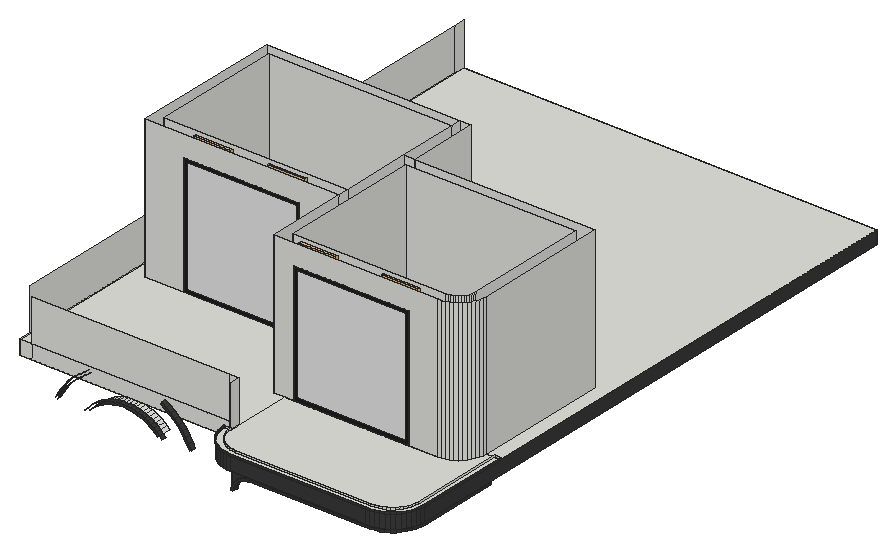
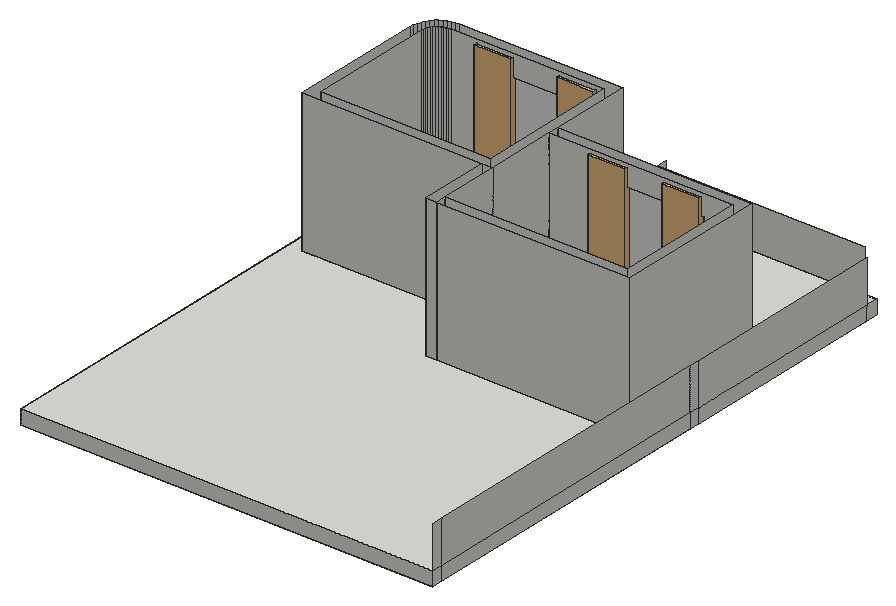
# SketchUp Ruby script. Lengths in inches.
U = 1.inch
M = Sketchup.active_model
def pt(a) = Geom::Point3d.new(a.map { |v| v * U })
def face(e, loops, mat)
  f = e.add_face(loops[0].map { |a| pt(a) })
  loops[1..].each { |l| e.add_face(l.map { |a| pt(a) }).erase! }
  f.material = f.back_material = mat if mat
  f
end
# faces: each face lists its corners as indices into pts; further lists are holes
def faces(e, pts, list, mat = nil) = list.each { |f| face(e, (f[0].is_a?(Array) ? f : [f]).map { |l| l.map { |i| pts[i] } }, mat) }
# xy, xz, yz: faces in a plane at the given z, y or x. An outline is a flat list of corners, or four numbers for a rectangle; further outlines are holes
def ring(l) = l.size == 4 ? [[l[0], l[1]], [l[2], l[1]], [l[2], l[3]], [l[0], l[3]]] : l.each_slice(2).to_a
def flat(e, list, mat, &to3) = list.each { |f| face(e, (f[0].is_a?(Array) ? f : [f]).map { |l| ring(l).map { |u, v| to3.(u, v) } }, mat) }
def xy(e, z, list, mat = nil) = flat(e, list, mat) { |x, y| [x, y, z] }
def xz(e, y, list, mat = nil) = flat(e, list, mat) { |x, z| [x, y, z] }
def yz(e, x, list, mat = nil) = flat(e, list, mat) { |y, z| [x, y, z] }
def lines(e, pts, list) = list.each { |a, b| e.add_line(pt(pts[a]), pt(pts[b])) }
# prism: a flat outline (further loops are holes) pulled along v
def prism(e, loops, v, mat = nil)
  f = face(e, loops, mat); d = Geom::Vector3d.new(v.map { |x| x * U })
  f.pushpull(f.normal.samedirection?(d) ? d.length : -d.length)
end
def box(e, o, s, mat = nil) = prism(e, [[o, [o[0] + s[0], o[1], o[2]], [o[0] + s[0], o[1] + s[1], o[2]], [o[0], o[1] + s[1], o[2]]]], [0, 0, s[2]], mat)
def at(x, y, z, deg = 0) = Geom::Transformation.translation(pt([x, y, z])) * Geom::Transformation.rotation(ORIGIN, Z_AXIS, deg.degrees)
def axes(o, x, y, z) = Geom::Transformation.new([*x, 0, *y, 0, *z, 0, *pt(o).to_a, 1])
def part(name) = M.definitions.add(name)
# library, detail: a bought-in or finely detailed component or shape, given as its bounding box
def library(name, o, s) = part(name).tap { |d| box(d.entities, o, s) }
def detail(e, o, s) = box(e.add_group.entities, o, s)
def put(e, d, t, mat = nil) = e.add_instance(d, t).tap { |i| i.material = mat if mat }
def group(e, t, mat = nil) = e.add_group.tap { |g| g.transformation = t; g.material = mat if mat }.entities
root = M.entities
M.materials.add("[Color M07]").color = [58, 58, 58]
M.materials.add("[Color M08]").color = [30, 30, 30]
M.materials.add("[Mirror 02]").color = [229, 229, 229]
c1 = library("Curtains 004",[-15.59,-2.26,0],[31.18,4.52,116.91])
xy(root,238.1,[[217.25,0,219.1875,4.75]])
xy(root,250.0625,[[233.71,0,233.71,4.75,331.6,4.75,334.94,4.79,338.01,5.25,340.98,6.125,343.8125,7.39,346.45,9.02,348.84,10.99,350.9375,13.27,352.71,15.82,354.125,18.57,355.16,21.5,355.78,24.53,356,27.76,356,96.75,360.75,96.75,360.75,27.6,360.5,23.89,359.74,20.22,358.5,16.69,356.79,13.36,354.65,10.29,352.11,7.54,349.22,5.15,346.04,3.18,342.625,1.65,339.03,0.6,335.33,0.05,331.63,0]],"[Color M07]")
xy(root,251.99,[[233.4,0,233.48,0.75]],"[Color M07]")
xy(root,252,[[216.6875,0.75,213.16,0.98,209.7,1.67,206.36,2.81,203.1875,4.37,200.25,6.33,197.6,8.66,195.27,11.3125,193.3,14.25,191.74,17.42,190.61,20.76,189.92,24.23,189.6875,27.75,189.99,24.2,190.75,20.73,191.95,17.375,193.57,14.21,195.58,11.27,197.96,8.625,200.66,6.3,203.63,4.35,206.83,2.79,210.21,1.67,213.7,0.98,217.25,0.75],[217.25,0.75,217.25,6.3,214.48,6.66,211.76,7.33,209.15,8.32,206.66,9.6,204.34,11.16,202.22,12.98,200.32,15.03,198.68,17.29,197.31,19.73,196.23,22.31,195.46,24.99,195,27.75,189.6875,27.75,189.99,24.2,190.75,20.73,191.95,17.375,193.57,14.21,195.58,11.27,197.96,8.625,200.66,6.3,203.63,4.35,206.83,2.79,210.21,1.67,213.7,0.98],[217.25,0.75,233.66,6.3],[[233.66,4.75,233.66,6.3,217.25,6.3,214.48,6.66,211.76,7.33,209.15,8.32,206.66,9.6,204.34,11.16,202.22,12.98,200.32,15.03,198.68,17.29,197.31,19.73,196.23,22.31,195.46,24.99,195,27.75,195,96.75,356,96.75,356,27.76,355.78,24.53,355.16,21.5,354.125,18.57,352.71,15.82,350.9375,13.27,348.84,10.99,346.45,9.02,343.8125,7.39,340.98,6.125,338.01,5.25,334.94,4.79,331.6,4.75],[208.88,75.77,344.63,81.77]],[9,36.75,9,498.75,351,498.75,351,105.75,186,105.75,186,36.75],
  [186,36.75,195,105.75],[195,96.75,351,105.75],[351,96.75,360,105.75],[351,105.75,360,507.75],[9,498.75,351,507.75]])
xy(root,252,[[233.66,0,233.72,0.75],[233.72,0,233.79,0.75],[233.79,0,234.52,0.75],[234.52,0,235.85,0.75],[235.85,0,331.63,0,331.625,0.75,235.85,0.75],
  [331.63,0,335.33,0.05,339.03,0.6,342.625,1.65,346.04,3.18,349.22,5.15,352.11,7.54,354.65,10.29,356.79,13.36,358.5,16.69,359.74,20.22,360.5,23.89,360.75,27.6,360,27.625,359.75,23.99,359.02,20.42,357.81,16.99,356.15,13.75,354.0625,10.76,351.59,8.08,348.79,5.76,345.69,3.84,342.36,2.36,338.87,1.34,335.27,0.8,331.625,0.75],[360.75,27.6,360.75,96.75,360,96.75,360,27.625]],"[Color M07]")
xy(root,255.1875,[[208.88,75.77,344.63,81.77]])
xy(root,264,[[216.6875,0.75,213.16,0.98,209.7,1.67,206.36,2.81,203.1875,4.37,200.25,6.33,197.6,8.66,195.27,11.3125,193.3,14.25,191.74,17.42,190.61,20.76,189.92,24.23,189.6875,27.75,195,27.75,195.1875,24.92,195.74,22.14,196.65,19.45,197.91,16.91,199.48,14.55,201.35,12.41,203.48,10.54,205.84,8.97,208.39,7.71,211.07,6.8,213.86,6.25,216.86,6.05,331.59,6.05,334.84,6.09,337.73,6.53,340.53,7.35,343.2,8.54,345.6875,10.08,347.94,11.94,349.92,14.09,351.59,16.49,352.93,19.09,353.9,21.85,354.49,24.71,354.7,27.8,354.7,108.42,360,108.42,360,27.625,359.75,23.99,359.02,20.42,357.81,16.99,356.15,13.75,354.0625,10.76,351.59,8.08,348.79,5.76,345.69,3.84,342.36,2.36,338.87,1.34,335.27,0.8,331.625,0.75],[216.86,6.05,331.59,6.05,334.84,6.09,337.73,6.53,340.53,7.35,343.2,8.54,345.6875,10.08,347.94,11.94,349.92,14.09,351.59,16.49,352.93,19.09,353.9,21.85,354.49,24.71,354.7,27.8,354.7,108.42,348,108.42,347.8,105.42,347.22,102.47,346.25,99.62,344.92,96.93,343.25,94.43,341.27,92.17,339.01,90.1875,336.51,88.52,333.82,87.1875,330.97,86.22,328.02,85.63,325.02,85.4375,195,85.4375,195,27.75,195.1875,24.92,195.74,22.14,196.65,19.45,197.91,16.91,199.48,14.55,201.35,12.41,203.48,10.54,205.84,8.97,208.39,7.71,211.07,6.8,213.86,6.25],[9,36.75,195,36.75,195,85.4375,185.6875,85.4375,185.6875,154.4375,21,154.4375,21,283.4375,194.6875,283.4375,194.6875,223.4375,348,223.4375,348,108.42,360,108.42,360,507.75,9,507.75],[185.6875,85.4375,185.6875,223.4375,348,223.4375,348,108.42,347.8,105.42,347.22,102.47,346.25,99.62,344.92,96.93,343.25,94.43,341.27,92.17,339.01,90.1875,336.51,88.52,333.82,87.1875,330.97,86.22,328.02,85.63,325.02,85.4375,300.68,85.4375,300.68,94.4375,325.02,94.4375,326.85,94.56,328.64,94.91,330.37,95.5,332.01,96.31,333.53,97.33,334.91,98.53,336.11,99.91,337.13,101.43,337.9375,103.07,338.52,104.8,338.88,106.59,339,108.42,339,214.4375,194.6875,214.4375,194.6875,94.4375,202.87,94.4375,202.87,85.4375],[202.87,87.8125,300.68,94.4375],
  [194.6875,94.4375,325.02,94.4375,326.85,94.56,328.64,94.91,330.37,95.5,332.01,96.31,333.53,97.33,334.91,98.53,336.11,99.91,337.13,101.43,337.9375,103.07,338.52,104.8,338.88,106.59,339,108.42,339,214.4375,194.6875,214.4375],[21,154.4375,21,283.4375,185.6875,283.4375,185.6875,274.4375,30,274.4375,30,163.4375,54.24,163.4375,54.24,154.4375],[152.05,154.4375,185.6875,163.4375],[54.24,156.8125,152.05,163.4375],[30,163.4375,185.6875,274.4375],
  [185.6875,223.4375,194.6875,283.4375]])
xy(root,264,[[216.67,0.3125,213.11,0.55,209.59,1.25,206.1875,2.4,202.97,3.99,199.98,5.98,197.29,8.35,194.92,11.05,192.93,14.03,191.34,17.25,190.18,20.65,189.48,24.17,189.25,27.72,189.6875,27.75,189.92,24.23,190.61,20.76,191.74,17.42,193.3,14.25,195.27,11.3125,197.6,8.66,200.25,6.33,203.1875,4.37,206.36,2.81,209.7,1.67,213.16,0.98,216.6875,0.75,331.625,0.75,335.27,0.8,338.87,1.34,342.36,2.36,345.69,3.84,348.79,5.76,351.59,8.08,354.0625,10.76,356.15,13.75,357.81,16.99,359.02,20.42,359.75,23.99,360,27.625,360,108.42,360.4375,108.42,360.4375,27.61,360.1875,23.93,359.44,20.31,358.21,16.82,356.52,13.52,354.4,10.49,351.89,7.77,349.04,5.41,345.9,3.46,342.52,1.95,338.96,0.91,335.3,0.36,331.63,0.3125]],"[Color M07]")
xy(root,264,[[202.87,85.4375,300.68,87.8125],[54.24,154.4375,152.05,156.8125]],"[Color M08]")
xz(root,0,[[217.25,238.1,219.1875,238.1,219.5625,239.64,220.16,241.24,220.93,242.76,221.875,244.18,222.98,245.48,224.22,246.65,225.6,247.66,227.07,248.51,228.64,249.18,230.28,249.67,231.96,249.96,233.71,250.0625,331.63,250.0625,331.63,252,233.66,252,233.48,251.99,233.4,251.99,233.3,251.98,233.18,251.97,232.69,251.94,231.9375,251.9,231.73,251.89,231.46,251.84,231.18,251.79,229.83,251.56,227.98,251,227.09,250.625,226.21,250.24,224.53,249.28,223.76,248.71,222.98,248.14,222.28,247.48,221.57,246.82,220.95,246.08,220.33,245.35,219.79,244.54,219.26,243.74,218.38,242.02,218.04,241.12,217.875,240.66,217.71,240.21,217.59,239.74,217.54,239.51,217.48,239.28,217.42,239.04,217.36,238.81,217.25,238.34]],"[Color M07]")
xz(root,0.3125,[[216.67,264,331.63,265.57]],"[Color M07]")
xz(root,0.75,[[217.25,238.34,217.36,238.81,217.42,239.04,217.48,239.28,217.54,239.51,217.59,239.74,217.71,240.21,217.875,240.66,218.04,241.12,218.38,242.02,219.26,243.74,219.79,244.54,220.33,245.35,220.95,246.08,221.57,246.82,222.28,247.48,222.98,248.14,223.76,248.71,224.53,249.28,226.21,250.24,227.09,250.625,227.98,251,229.83,251.56,231.18,251.79,231.46,251.84,231.73,251.89,231.9375,251.9,232.69,251.94,233.18,251.97,233.3,251.98,233.4,251.99,233.48,251.99,233.66,252,217.25,252],[216.6875,252,331.625,264]],"[Color M07]")
xz(root,4.75,[[217.25,238.1,217.25,238.34,217.71,240.21,218.38,242.02,219.26,243.74,220.33,245.35,221.57,246.82,222.98,248.14,224.53,249.28,226.21,250.24,227.98,251,229.83,251.56,231.73,251.89,233.66,252,331.6,252,331.6,250.0625,233.71,250.0625,231.96,249.96,230.28,249.67,228.64,249.18,227.07,248.51,225.6,247.66,224.22,246.65,222.98,245.48,221.875,244.18,220.93,242.76,220.16,241.24,219.5625,239.64,219.1875,238.1]],"[Color M07]")
xz(root,6.05,[[216.86,264,331.59,265.57]])
xz(root,6.3,[[217.25,238.34,217.25,252,233.66,252,231.73,251.89,229.83,251.56,227.98,251,226.21,250.24,224.53,249.28,222.98,248.14,221.57,246.82,220.33,245.35,219.26,243.74,218.38,242.02,217.71,240.21]])
xz(root,27.75,[[189.6875,252,195,264],[189.6875,264,195,265.57]])
xz(root,36.75,[[9,252,18.96,264],[18.96,252,186,264],[186,252,195,264],[18.96,264,186,300],[186,264,195,300]])
xz(root,75.77,[[208.88,252,344.63,255.1875]])
xz(root,81.77,[[208.88,252,344.63,255.1875]])
xz(root,85.4375,[[185.6875,264,202.87,264,202.87,366.4375,300.68,366.4375,300.68,264,325.02,264,325.02,384,185.6875,384]])
xz(root,85.4375,[[[202.87,264,300.68,366.4375],[205.38,266.52,298.16,363.92]]],"[Color M08]")
xz(root,87.8125,[[202.87,264,300.68,366.4375]],"[Mirror 02]")
xz(root,94.4375,[[194.6875,264,194.6875,384,325.02,384,325.02,264,300.68,264,300.68,366.4375,202.87,366.4375,202.87,264]])
xz(root,96.75,[[360,250.0625,360.75,252]])
xz(root,108.42,[[354.7,264,360.4375,265.57]])
xz(root,154.4375,[[21,264,54.24,264,54.24,366.4375,152.05,366.4375,152.05,264,185.6875,264,185.6875,384,21,384]])
xz(root,154.4375,[[[54.24,264,152.05,366.4375],[56.75,266.52,149.53,363.92]]],"[Color M08]")
xz(root,156.8125,[[54.24,264,152.05,366.4375]],"[Mirror 02]")
xz(root,163.4375,[[30,264,30,384,185.6875,384,185.6875,264,152.05,264,152.05,366.4375,54.24,366.4375,54.24,264]])
xz(root,214.4375,[[194.6875,264,339,384]])
xz(root,223.4375,[[185.6875,264,194.6875,384],[194.6875,264,348,384]])
xz(root,274.4375,[[30,264,185.6875,384]])
xz(root,283.4375,[[21,264,185.6875,384],[185.6875,264,194.6875,384]])
xz(root,507.75,[[9,252,360,264]])
yz(root,9,[[36.75,252,46.71,264],[46.71,252,225.75,264],[225.75,252,234.75,264],[234.75,252,498.75,264],[498.75,252,507.75,264],
  [46.71,264,225.75,300],[225.75,264,234.75,300],[234.75,264,498.75,300],[498.75,264,507.75,300]])
yz(root,21,[[154.4375,264,283.4375,384]])
yz(root,30,[[163.4375,264,274.4375,384]])
yz(root,54.24,[[156.8125,264,163.4375,366.4375]])
yz(root,54.24,[[154.4375,264,156.8125,366.4375]],"[Color M08]")
yz(root,152.05,[[156.8125,264,163.4375,366.4375]])
yz(root,152.05,[[154.4375,264,156.8125,366.4375]],"[Color M08]")
yz(root,185.6875,[[85.4375,264,154.4375,384],[154.4375,264,163.4375,384],[163.4375,264,223.4375,384],[223.4375,264,274.4375,384],[274.4375,264,283.4375,384]])
yz(root,194.6875,[[94.4375,264,214.4375,384],[223.4375,264,283.4375,384]])
yz(root,195,[[27.75,252,36.75,264],[27.75,264,36.75,300]])
yz(root,202.87,[[87.8125,264,94.4375,366.4375]])
yz(root,202.87,[[85.4375,264,87.8125,366.4375]],"[Color M08]")
yz(root,208.88,[[75.77,252,81.77,255.1875]])
yz(root,217.25,[[0.75,238.34,6.3,252]])
yz(root,217.25,[[0,238.1,0.75,238.34]],"[Color M07]")
yz(root,300.68,[[87.8125,264,94.4375,366.4375]])
yz(root,300.68,[[85.4375,264,87.8125,366.4375]],"[Color M08]")
yz(root,339,[[108.42,264,214.4375,384]])
yz(root,344.63,[[75.77,252,81.77,255.1875]])
yz(root,348,[[108.42,264,223.4375,384]])
yz(root,354.7,[[27.8,264,108.42,265.57]])
yz(root,356,[[27.76,250.0625,96.75,252]],"[Color M07]")
yz(root,360,[[27.625,252,507.75,264]],"[Color M07]")
yz(root,360.4375,[[27.61,264,108.42,265.57]],"[Color M07]")
yz(root,360.75,[[27.6,250.0625,96.75,252]],"[Color M07]")
p = [[219.1875,0,238.1],[219.1875,4.75,238.1],[219.5625,4.75,239.64],[219.5625,0,239.64],[217.36,0,238.81],[217.36,0.75,238.81],
  [217.25,0.75,238.34],[217.25,0,238.34],[217.25,4.75,238.34],[217.25,6.3,238.34],[217.71,6.3,240.21],[217.71,4.75,240.21],
  [50.83,27.75,238.37],[52.99,27.75,242.52],[52.99,24.0625,242.52],[50.83,24.0625,238.37],[160.97,27.75,242.52],[163.125,27.75,238.37],
  [163.125,24.0625,238.37],[160.97,24.0625,242.52],[76.46,27.75,241.05],[74.4,27.75,238.74],[74.4,24.0625,238.74],[76.46,24.0625,241.05],
  [139.5625,27.75,238.74],[137.5,27.75,241.05],[137.5,24.0625,241.05],[139.5625,24.0625,238.74],[217.42,0,239.04],[217.42,0.75,239.04],
  [217.48,0,239.28],[217.48,0.75,239.28],[51.2,27.75,243.53],[48.97,27.75,239.25],[48.97,24.0625,239.25],[51.2,24.0625,243.53],
  [164.99,27.75,239.25],[162.76,27.75,243.53],[162.76,24.0625,243.53],[164.99,24.0625,239.25],[217.54,0,239.51],[217.54,0.75,239.51],
  [217.59,0,239.74],[217.59,0.75,239.74],[220.16,4.75,241.24],[220.16,0,241.24],[77.95,24.0625,239.625],[77.95,27.75,239.625],
  [80.0625,27.75,241.68],[80.0625,24.0625,241.68],[133.89,24.0625,241.68],[133.89,27.75,241.68],[136.01,27.75,239.625],[136.01,24.0625,239.625],
  [80.0625,29.9375,241.68],[77.95,29.9375,239.625],[136.01,29.9375,239.625],[133.89,29.9375,241.68],[80.0625,36.75,241.68],[77.95,36.75,239.625],
  [136.01,36.75,239.625],[133.89,36.75,241.68],[217.71,0,240.21],[217.71,0.75,240.21],[217.875,0,240.66],[217.875,0.75,240.66],
  [218.38,6.3,242.02],[218.38,4.75,242.02],[218.04,0,241.12],[218.04,0.75,241.12],[218.38,0,242.02],[218.38,0.75,242.02],
  [78.6875,27.75,243.21],[78.6875,24.0625,243.21],[135.27,27.75,243.21],[135.27,24.0625,243.21],[220.93,4.75,242.76],[220.93,0,242.76],
  [82.33,27.75,243.57],[82.33,24.0625,243.57],[131.63,24.0625,243.57],[131.63,27.75,243.57],[82.33,29.9375,243.57],[131.63,29.9375,243.57],
  [82.33,36.75,243.57],[131.63,36.75,243.57],[218.82,0,242.88],[218.82,0.75,242.88],[219.26,6.3,243.74],[219.26,4.75,243.74],
  [55.45,27.75,246.49],[55.45,24.0625,246.49],[158.51,27.75,246.49],[158.51,24.0625,246.49],[221.875,4.75,244.18],[221.875,0,244.18],
  [219.26,0,243.74],[219.26,0.75,243.74],[81.0625,27.75,245.19],[81.0625,24.0625,245.19],[132.89,27.75,245.19],[132.89,24.0625,245.19],
  [53.74,27.75,247.64],[53.74,24.0625,247.64],[160.22,27.75,247.64],[160.22,24.0625,247.64],[84.72,27.75,245.28],[84.72,24.0625,245.28],
  [129.24,24.0625,245.28],[129.24,27.75,245.28],[84.72,29.9375,245.28],[129.24,29.9375,245.28],[84.72,36.75,245.28],[129.24,36.75,245.28],
  [219.79,0,244.54],[219.79,0.75,244.54],[220.33,6.3,245.35],[220.33,4.75,245.35],[222.98,4.75,245.48],[222.98,0,245.48],
  [220.33,0,245.35],[220.33,0.75,245.35],[83.58,27.75,247],[83.58,24.0625,247],[130.38,27.75,247],[130.38,24.0625,247],
  [220.95,0,246.08],[220.95,0.75,246.08],[221.57,6.3,246.82],[221.57,4.75,246.82],[87.23,27.75,246.82],[87.23,24.0625,246.82],
  [126.72,24.0625,246.82],[126.72,27.75,246.82],[87.23,29.9375,246.82],[126.72,29.9375,246.82],[87.23,36.75,246.82],[126.72,36.75,246.82],
  [224.22,4.75,246.65],[224.22,0,246.65],[221.57,0,246.82],[221.57,0.75,246.82],[58.2,27.75,250.27],[58.2,24.0625,250.27],
  [155.76,27.75,250.27],[155.76,24.0625,250.27],[225.6,4.75,247.66],[225.6,0,247.66],[222.28,0,247.48],[222.28,0.75,247.48],
  [222.98,6.3,248.14],[222.98,4.75,248.14],[89.85,27.75,248.17],[89.85,24.0625,248.17],[124.1,24.0625,248.17],[124.1,27.75,248.17],
  [89.85,29.9375,248.17],[124.1,29.9375,248.17],[89.85,36.75,248.17],[124.1,36.75,248.17],[86.22,27.75,248.62],[86.22,24.0625,248.62],
  [127.74,27.75,248.62],[127.74,24.0625,248.62],[222.98,0,248.14],[222.98,0.75,248.14],[56.58,27.75,251.54],[56.58,24.0625,251.54],
  [157.375,27.75,251.54],[157.375,24.0625,251.54],[227.07,4.75,248.51],[227.07,0,248.51],[223.76,0,248.71],[223.76,0.75,248.71],
  [224.53,6.3,249.28],[224.53,4.75,249.28],[92.57,27.75,249.33],[92.57,24.0625,249.33],[121.39,24.0625,249.33],[121.39,27.75,249.33],
  [92.57,29.9375,249.33],[121.39,29.9375,249.33],[92.57,36.75,249.33],[121.39,36.75,249.33],[228.64,4.75,249.18],[228.64,0,249.18],
  [88.98,27.75,250.04],[88.98,24.0625,250.04],[124.98,27.75,250.04],[124.98,24.0625,250.04],[224.53,0,249.28],[224.53,0.75,249.28],
  [230.28,4.75,249.67],[230.28,0,249.67],[225.37,0,249.76],[225.37,0.75,249.76],[226.21,6.3,250.24],[226.21,4.75,250.24],
  [95.35,27.75,250.28],[95.35,24.0625,250.28],[118.6,24.0625,250.28],[118.6,27.75,250.28],[95.35,29.9375,250.28],[118.6,29.9375,250.28],
  [95.35,36.75,250.28],[118.6,36.75,250.28],[231.96,4.75,249.96],[231.96,0,249.96],[226.21,0,250.24],[226.21,0.75,250.24],
  [233.71,4.75,250.0625],[233.71,0,250.0625],[91.83,27.75,251.25],[91.83,24.0625,251.25],[122.13,27.75,251.25],[122.13,24.0625,251.25],
  [331.63,0,252],[331.63,0,250.0625],[335.33,0.05,250.0625],[335.33,0.05,252],[339.03,0.6,250.0625],[339.03,0.6,252],
  [342.625,1.65,250.0625],[342.625,1.65,252],[346.04,3.18,250.0625],[346.04,3.18,252],[349.22,5.15,250.0625],[349.22,5.15,252],
  [331.6,4.75,250.0625],[331.6,4.75,252],[334.94,4.79,252],[334.94,4.79,250.0625],[338.01,5.25,252],[338.01,5.25,250.0625],
  [352.11,7.54,250.0625],[352.11,7.54,252],[340.98,6.125,252],[340.98,6.125,250.0625],[343.8125,7.39,252],[343.8125,7.39,250.0625],
  [346.45,9.02,252],[346.45,9.02,250.0625],[354.65,10.29,250.0625],[354.65,10.29,252],[348.84,10.99,252],[348.84,10.99,250.0625],
  [356.79,13.36,250.0625],[356.79,13.36,252],[350.9375,13.27,252],[350.9375,13.27,250.0625],[352.71,15.82,252],[352.71,15.82,250.0625],
  [358.5,16.69,250.0625],[358.5,16.69,252],[354.125,18.57,252],[354.125,18.57,250.0625],[359.74,20.22,250.0625],[359.74,20.22,252],
  [355.16,21.5,252],[355.16,21.5,250.0625],[360.5,23.89,250.0625],[360.5,23.89,252],[355.78,24.53,252],[355.78,24.53,250.0625],
  [360.75,27.6,250.0625],[360.75,27.6,252],[356,27.76,252],[356,27.76,250.0625],[227.09,0,250.625],[227.09,0.75,250.625],
  [227.98,6.3,251],[227.98,4.75,251],[61.23,27.75,253.83],[61.23,24.0625,253.83],[98.21,27.75,251.03],[98.21,24.0625,251.03],
  [115.75,24.0625,251.03],[115.75,27.75,251.03],[152.73,27.75,253.83],[152.73,24.0625,253.83],[98.21,29.9375,251.03],[115.75,29.9375,251.03],
  [98.21,36.75,251.03],[115.75,36.75,251.03],[227.98,0,251],[227.98,0.75,251],[229.83,0,251.56],[229.83,0.75,251.56],
  [229.83,6.3,251.56],[229.83,4.75,251.56],[101.1,27.75,251.57],[101.1,24.0625,251.57],[112.85,24.0625,251.57],[112.85,27.75,251.57],
  [101.1,29.9375,251.57],[112.85,29.9375,251.57],[101.1,36.75,251.57],[112.85,36.75,251.57],[94.76,27.75,252.26],[94.76,24.0625,252.26],
  [119.2,27.75,252.26],[119.2,24.0625,252.26],[59.71,27.75,255.22],[59.71,24.0625,255.22],[154.25,27.75,255.22],[154.25,24.0625,255.22],
  [231.18,0,251.79],[231.18,0.75,251.79],[231.73,6.3,251.89],[231.73,4.75,251.89],[104.03,27.75,251.89],[104.03,24.0625,251.89],
  [109.92,24.0625,251.89],[109.92,27.75,251.89],[104.03,29.9375,251.89],[109.92,29.9375,251.89],[104.03,36.75,251.89],[109.92,36.75,251.89],
  [231.46,0,251.84],[231.46,0.75,251.84],[231.73,0,251.89],[231.73,0.75,251.89],[231.9375,0,251.9],[231.9375,0.75,251.9],
  [232.69,0,251.94],[232.69,0.75,251.94],[233.18,0,251.97],[233.18,0.75,251.97],[233.66,6.3,252],[233.66,4.75,252],
  [105.32,27.75,251.9375],[105.32,26.6875,251.9375],[106.98,26.6875,252],[106.98,24.0625,252],[108.92,26.6875,251.93],[108.92,27.75,251.93],
  [106.98,27.75,252],[106.98,29.9375,252],[106.98,36.75,252],[233.3,0,251.98],[233.3,0.75,251.98],[233.4,0,251.99],
  [233.4,0.75,251.99],[233.66,0,252],[233.66,0.75,252],[233.48,0.75,251.99],[233.48,0,251.99],[216.6875,0.75,264],
  [213.16,0.98,264],[213.16,0.98,252],[216.6875,0.75,252],[335.27,0.8,264],[331.625,0.75,264],[331.625,0.75,252],
  [335.27,0.8,252],[338.87,1.34,264],[338.87,1.34,252],[209.7,1.67,264],[209.7,1.67,252],[342.36,2.36,264],
  [342.36,2.36,252],[206.36,2.81,264],[206.36,2.81,252],[345.69,3.84,264],[345.69,3.84,252],[203.1875,4.37,264],
  [203.1875,4.37,252],[348.79,5.76,264],[348.79,5.76,252],[200.25,6.33,264],[200.25,6.33,252],[351.59,8.08,264],
  [351.59,8.08,252],[197.6,8.66,264],[197.6,8.66,252],[354.0625,10.76,264],[354.0625,10.76,252],[195.27,11.3125,264],
  [195.27,11.3125,252],[356.15,13.75,264],[356.15,13.75,252],[193.3,14.25,264],[193.3,14.25,252],[357.81,16.99,264],
  [357.81,16.99,252],[191.74,17.42,264],[191.74,17.42,252],[359.02,20.42,264],[359.02,20.42,252],[190.61,20.76,264],
  [190.61,20.76,252],[359.75,23.99,264],[359.75,23.99,252],[189.92,24.23,264],[189.92,24.23,252],[360,27.625,264],
  [360,27.625,252],[189.6875,27.75,264],[189.6875,27.75,252],[97.76,27.75,253.04],[97.76,24.0625,253.04],[116.2,27.75,253.04],
  [116.2,24.0625,253.04],[100.8,27.75,253.61],[100.8,24.0625,253.61],[113.16,27.75,253.61],[113.16,24.0625,253.61],[103.88,27.75,253.95],
  [103.88,24.0625,253.95],[110.08,27.75,253.95],[110.08,24.0625,253.95],[64.52,27.75,257.15],[64.52,24.0625,257.15],[149.44,27.75,257.15],
  [149.44,24.0625,257.15],[106.98,27.75,254.0625],[106.98,24.0625,254.0625],[63.11,27.75,258.66],[63.11,24.0625,258.66],[150.85,27.75,258.66],
  [150.85,24.0625,258.66],[68.05,27.75,260.22],[68.05,24.0625,260.22],[145.91,27.75,260.22],[145.91,24.0625,260.22],[66.75,27.75,261.82],
  [66.75,24.0625,261.82],[147.2,27.75,261.82],[147.2,24.0625,261.82],[71.8,27.75,263.01],[71.8,24.0625,263.01],[142.16,27.75,263.01],
  [142.16,24.0625,263.01],[70.63,27.75,264.71],[70.63,24.0625,264.71],[143.33,27.75,264.71],[143.33,24.0625,264.71],[75.74,27.75,265.51],
  [75.74,24.0625,265.51],[138.21,27.75,265.51],[138.21,24.0625,265.51],[213.11,0.55,265.57],[213.11,0.55,264],[216.67,0.3125,264],
  [216.67,0.3125,265.57],[331.63,0.3125,265.57],[331.63,0.3125,264],[335.3,0.36,264],[335.3,0.36,265.57],[338.96,0.91,264],
  [338.96,0.91,265.57],[209.59,1.25,265.57],[209.59,1.25,264],[342.52,1.95,264],[342.52,1.95,265.57],[206.1875,2.4,265.57],
  [206.1875,2.4,264],[345.9,3.46,264],[345.9,3.46,265.57],[202.97,3.99,265.57],[202.97,3.99,264],[349.04,5.41,264],
  [349.04,5.41,265.57],[199.98,5.98,265.57],[199.98,5.98,264],[351.89,7.77,264],[351.89,7.77,265.57],[197.29,8.35,265.57],
  [197.29,8.35,264],[213.86,6.25,264],[213.86,6.25,265.57],[216.86,6.05,265.57],[216.86,6.05,264],[331.59,6.05,264],
  [331.59,6.05,265.57],[334.84,6.09,265.57],[334.84,6.09,264],[337.73,6.53,265.57],[337.73,6.53,264],[211.07,6.8,264],
  [211.07,6.8,265.57],[340.53,7.35,265.57],[340.53,7.35,264],[208.39,7.71,264],[208.39,7.71,265.57],[343.2,8.54,265.57],
  [343.2,8.54,264],[205.84,8.97,264],[205.84,8.97,265.57],[354.4,10.49,264],[354.4,10.49,265.57],[194.92,11.05,265.57],
  [194.92,11.05,264],[345.6875,10.08,265.57],[345.6875,10.08,264],[203.48,10.54,264],[203.48,10.54,265.57],[347.94,11.94,265.57],
  [347.94,11.94,264],[201.35,12.41,264],[201.35,12.41,265.57],[356.52,13.52,264],[356.52,13.52,265.57],[192.93,14.03,265.57],
  [192.93,14.03,264],[349.92,14.09,265.57],[349.92,14.09,264],[199.48,14.55,264],[199.48,14.55,265.57],[358.21,16.82,264],
  [358.21,16.82,265.57],[191.34,17.25,265.57],[191.34,17.25,264],[351.59,16.49,265.57],[351.59,16.49,264],[197.91,16.91,264],
  [197.91,16.91,265.57],[352.93,19.09,265.57],[352.93,19.09,264],[359.44,20.31,264],[359.44,20.31,265.57],[196.65,19.45,264],
  [196.65,19.45,265.57],[190.18,20.65,265.57],[190.18,20.65,264],[353.9,21.85,265.57],[353.9,21.85,264],[195.74,22.14,264],
  [195.74,22.14,265.57],[360.1875,23.93,264],[360.1875,23.93,265.57],[189.48,24.17,265.57],[189.48,24.17,264],[354.49,24.71,265.57],
  [354.49,24.71,264],[195.1875,24.92,264],[195.1875,24.92,265.57],[360.4375,27.61,264],[360.4375,27.61,265.57],[189.25,27.72,265.57],
  [189.25,27.72,264],[354.7,27.8,265.57],[354.7,27.8,264],[195,27.75,264],[195,27.75,265.57],[189.6875,27.75,265.57],
  [194.98,28.1,265.57],[194.98,28.1,264],[325.02,85.4375,264],[328.02,85.63,264],[328.02,85.63,384],[325.02,85.4375,384],
  [330.97,86.22,264],[330.97,86.22,384],[333.82,87.1875,264],[333.82,87.1875,384],[336.51,88.52,264],[336.51,88.52,384],
  [339.01,90.1875,264],[339.01,90.1875,384],[339,90.18,384],[341.27,92.17,264],[341.27,92.17,384],[340.35,91.36,384],
  [343.25,94.43,264],[343.25,94.43,384],[326.85,94.56,264],[325.02,94.4375,264],[325.02,94.4375,384],[326.85,94.56,384],
  [344.92,96.93,264],[344.92,96.93,384],[328.64,94.91,264],[328.64,94.91,384],[330.37,95.5,264],[330.37,95.5,384],
  [332.01,96.31,264],[332.01,96.31,384],[333.53,97.33,264],[333.53,97.33,384],[346.25,99.62,264],[346.25,99.62,384],
  [345.58,98.26,384],[334.91,98.53,264],[334.91,98.53,384],[336.11,99.91,264],[336.11,99.91,384],[347.22,102.47,264],
  [347.22,102.47,384],[337.13,101.43,264],[337.13,101.43,384],[337.9375,103.07,264],[337.9375,103.07,384],[347.8,105.42,264],
  [347.8,105.42,384],[338.52,104.8,264],[338.52,104.8,384],[338.88,106.59,264],[338.88,106.59,384],[348,108.42,264],
  [348,108.42,384],[339,108.42,264],[339,108.42,384],[74.71,27.75,267.29],[74.71,24.0625,267.29],[139.25,27.75,267.29],
  [139.25,24.0625,267.29]]
faces(root,p,[[0,1,2,3],[4,5,6,7],[8,9,10,11],[12,13,14,15],[16,17,18,19],[20,21,22,23],[24,25,26,27],[28,29,5,4],
  [30,31,29,28],[32,33,34,35],[36,37,38,39],[31,30,40,41],[41,40,42,43],[3,2,44,45],[46,47,48,49],[50,51,52,53],
  [54,55,47,48],[56,57,51,52],[43,42,62,63],[63,62,64,65],[11,10,66,67],[65,64,68,69],[69,68,70,71],[72,20,23,73],
  [25,74,75,26],[45,44,76,77],[49,48,78,79],[80,81,51,50],[82,54,48,78],[57,83,81,51],[71,70,86,87],[67,66,88,89],
  [13,90,91,14],[92,16,19,93],[77,76,94,95],[87,86,96,97],[98,72,73,99],[74,100,101,75],[102,32,35,103],[37,104,105,38],
  [79,78,106,107],[108,109,81,80],[110,82,78,106],[83,111,109,81],[97,96,114,115],[89,88,116,117],[95,94,118,119],[115,114,120,121],
  [122,98,99,123],[100,124,125,101],[121,120,126,127],[117,116,128,129],[107,106,130,131],[132,133,109,108],[134,110,106,130],[111,135,133,109],
  [119,118,138,139],[127,126,140,141],[90,142,143,91],[144,92,93,145],[139,138,146,147],[141,140,148,149],[129,128,150,151],[131,130,152,153],
  [154,155,133,132],[156,134,130,152],[135,157,155,133],[160,122,123,161],[124,162,163,125],[149,148,164,165],[166,102,103,167],[104,168,169,105],
  [147,146,170,171],[165,164,172,173],[151,150,174,175],[153,152,176,177],[178,179,155,154],[180,156,152,176],[157,181,179,155],[171,170,184,185],
  [186,160,161,187],[162,188,189,163],[173,172,190,191],[185,184,192,193],[191,190,194,195],[175,174,196,197],[177,176,198,199],[200,201,179,178],
  [202,180,176,198],[181,203,201,179],[193,192,206,207],[195,194,208,209],[207,206,210,211],[212,186,187,213],[188,214,215,189],[216,217,218,219],
  [219,218,220,221],[221,220,222,223],[223,222,224,225],[225,224,226,227],[228,229,230,231],[231,230,232,233],[227,226,234,235],[233,232,236,237],
  [237,236,238,239],[239,238,240,241],[235,234,242,243],[241,240,244,245],[243,242,246,247],[245,244,248,249],[249,248,250,251],[247,246,252,253],
  [251,250,254,255],[253,252,256,257],[255,254,258,259],[257,256,260,261],[259,258,262,263],[261,260,264,265],[263,262,266,267],[209,208,268,269],
  [197,196,270,271],[142,272,273,143],[199,198,274,275],[276,277,201,200],[278,144,145,279],[280,202,198,274],[203,281,277,201],[269,268,284,285],
  [285,284,286,287],[271,270,288,289],[275,274,290,291],[292,293,277,276],[294,280,274,290],[281,295,293,277],[298,212,213,299],[214,300,301,215],
  [302,166,167,303],[168,304,305,169],[287,286,306,307],[289,288,308,309],[291,290,310,311],[312,313,293,292],[314,294,290,310],[295,315,313,293],
  [318,319,307,306],[320,321,319,318],[321,320,322,323],[323,322,324,325],[326,327,325,324],[309,308,328,329],[311,310,330,331,332,333],[334,335,313,312,333,332],
  [337,314,310,330,336],[315,337,336,335,313],[339,340,327,326],[341,342,340,339],[343,344,345,346],[347,348,349,350],[351,352,353,354],[355,351,354,356],
  [348,357,358,349],[359,355,356,360],[357,361,362,358],[363,359,360,364],[361,365,366,362],[367,363,364,368],[365,369,370,366],[371,367,368,372],
  [369,373,374,370],[375,371,372,376],[373,377,378,374],[379,375,376,380],[377,381,382,378],[383,379,380,384],[381,385,386,382],[387,383,384,388],
  [385,389,390,386],[391,387,388,392],[389,393,394,390],[395,391,392,396],[393,397,398,394],[399,298,299,400],[300,401,402,301],[403,399,400,404],
  [401,405,406,402],[407,403,404,408],[405,409,410,406],[272,411,412,273],[413,278,279,414],[415,407,408,416],[409,415,416,410],[417,302,303,418],
  [304,419,420,305],[411,421,422,412],[423,413,414,424],[425,417,418,426],[419,427,428,420],[421,429,430,422],[431,423,424,432],[433,425,426,434],
  [427,435,436,428],[429,437,438,430],[439,431,432,440],[441,442,443,444],[445,446,447,448],[448,447,449,450],[451,452,442,441],[450,449,453,454],
  [455,456,452,451],[454,453,457,458],[459,460,456,455],[458,457,461,462],[463,464,460,459],[462,461,465,466],[467,468,464,463],[466,465,489,490],
  [491,492,468,467],[490,489,501,502],[503,504,492,491],[502,501,509,510],[511,512,504,503],[510,509,519,520],[523,524,512,511],[520,519,529,530],
  [531,532,524,523],[530,529,537,538],[539,540,532,531],[603,433,434,604],[435,605,606,436]],"[Color M07]")
faces(root,p,[[58,54,55,59],[60,56,57,61],[84,82,54,58],[61,57,83,85],[112,110,82,84],[85,83,111,113],[136,134,110,112],[113,111,135,137],
  [158,156,134,136],[137,135,157,159],[182,180,156,158],[159,157,181,183],[204,202,180,182],[183,181,203,205],[282,280,202,204],[205,203,281,283],
  [296,294,280,282],[283,281,295,297],[316,314,294,296],[297,295,315,317],[330,336,332,331],[336,335,334,332],[338,337,314,316],[317,315,337,338],
  [469,470,471,472],[473,474,475,476],[476,475,477,478],[479,480,470,469],[478,477,481,482],[483,484,480,479],[482,481,485,486],[487,488,484,483],
  [486,485,493,494],[495,496,488,487],[494,493,497,498],[499,500,496,495],[498,497,505,506],[507,508,500,499],[506,505,513,514],[515,516,508,507],
  [514,513,517,518],[521,522,516,515],[518,517,525,526],[527,528,522,521],[526,525,533,534],[535,536,528,527],[534,533,541,542],[535,543,544,536],
  [539,545,397,540],[546,544,543,547],[548,549,550,551],[549,552,553,550],[552,554,555,553],[554,556,557,555],[556,558,559,560,557],[558,561,562,563,559],
  [561,564,565,562],[566,567,568,569],[564,570,571,565],[572,566,569,573],[574,572,573,575],[576,574,575,577],[578,576,577,579],[570,580,581,582,571],
  [583,578,579,584],[585,583,584,586],[580,587,588,581],[589,585,586,590],[591,589,590,592],[587,593,594,588],[595,591,592,596],[597,595,596,598],
  [593,599,600,594],[601,597,598,602]])
put(root,c1,at(287.26,94.4375,264))
put(root,c1,at(217.29,94.4375,264))
put(root,c1,at(135.42,163.4375,264))
put(root,c1,at(72.67,163.4375,264))
